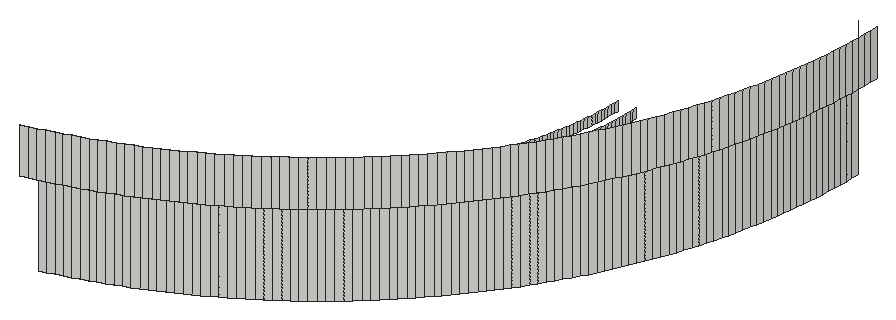
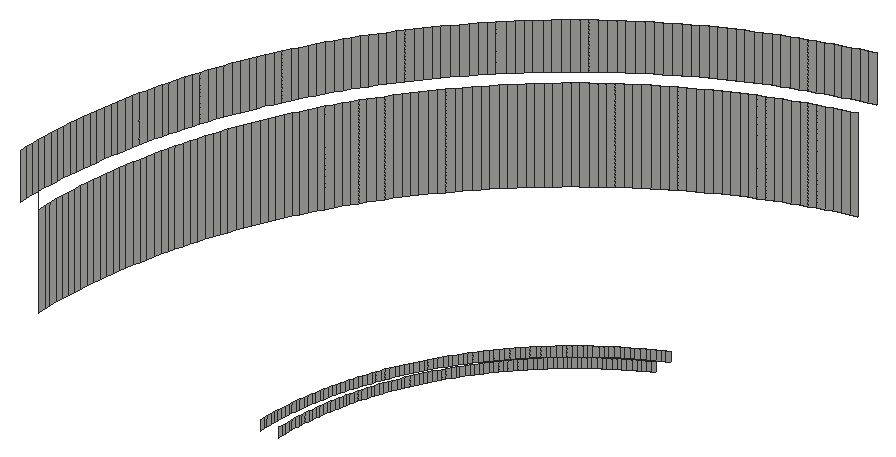
# SketchUp Ruby script. Lengths in inches.
U = 1.inch
M = Sketchup.active_model
def pt(a) = Geom::Point3d.new(a.map { |v| v * U })
def face(e, loops, mat)
  f = e.add_face(loops[0].map { |a| pt(a) })
  loops[1..].each { |l| e.add_face(l.map { |a| pt(a) }).erase! }
  f.material = f.back_material = mat if mat
  f
end
# faces: each face lists its corners as indices into pts; further lists are holes
def faces(e, pts, list, mat = nil) = list.each { |f| face(e, (f[0].is_a?(Array) ? f : [f]).map { |l| l.map { |i| pts[i] } }, mat) }
# xy, xz, yz: faces in a plane at the given z, y or x. An outline is a flat list of corners, or four numbers for a rectangle; further outlines are holes
def ring(l) = l.size == 4 ? [[l[0], l[1]], [l[2], l[1]], [l[2], l[3]], [l[0], l[3]]] : l.each_slice(2).to_a
def flat(e, list, mat, &to3) = list.each { |f| face(e, (f[0].is_a?(Array) ? f : [f]).map { |l| ring(l).map { |u, v| to3.(u, v) } }, mat) }
def xy(e, z, list, mat = nil) = flat(e, list, mat) { |x, y| [x, y, z] }
def xz(e, y, list, mat = nil) = flat(e, list, mat) { |x, z| [x, y, z] }
def yz(e, x, list, mat = nil) = flat(e, list, mat) { |y, z| [x, y, z] }
def lines(e, pts, list) = list.each { |a, b| e.add_line(pt(pts[a]), pt(pts[b])) }
# prism: a flat outline (further loops are holes) pulled along v
def prism(e, loops, v, mat = nil)
  f = face(e, loops, mat); d = Geom::Vector3d.new(v.map { |x| x * U })
  f.pushpull(f.normal.samedirection?(d) ? d.length : -d.length)
end
def box(e, o, s, mat = nil) = prism(e, [[o, [o[0] + s[0], o[1], o[2]], [o[0] + s[0], o[1] + s[1], o[2]], [o[0], o[1] + s[1], o[2]]]], [0, 0, s[2]], mat)
def at(x, y, z, deg = 0) = Geom::Transformation.translation(pt([x, y, z])) * Geom::Transformation.rotation(ORIGIN, Z_AXIS, deg.degrees)
def axes(o, x, y, z) = Geom::Transformation.new([*x, 0, *y, 0, *z, 0, *pt(o).to_a, 1])
def part(name) = M.definitions.add(name)
# library, detail: a bought-in or finely detailed component or shape, given as its bounding box
def library(name, o, s) = part(name).tap { |d| box(d.entities, o, s) }
def detail(e, o, s) = box(e.add_group.entities, o, s)
def put(e, d, t, mat = nil) = e.add_instance(d, t).tap { |i| i.material = mat if mat }
def group(e, t, mat = nil) = e.add_group.tap { |g| g.transformation = t; g.material = mat if mat }.entities
root = M.entities
yz(root,285.99,[[233.37,348,233.58,348.5]])
yz(root,286,[[233.79,348,234,348.5]])
yz(root,286.99,[[233.33,348,233.55,348.5]])
yz(root,287,[[233.78,348,234,348.5]])
yz(root,299,[[233.62,349.5,234,354.5]])
yz(root,300,[[233.61,354.5,234,357]])
p = [[277.32,218.66,348],[277.12,218.5625,348],[277.12,218.5625,348.5],[277.32,218.66,348.5],[277.52,218.75,348],[277.52,218.75,348.5],
  [277.72,218.85,348],[277.72,218.85,348.5],[277.92,218.96,348],[277.92,218.96,348.5],[278.11,219.06,348],[278.11,219.06,348.5],
  [278.31,219.17,348],[278.31,219.17,348.5],[278.5,219.28,348],[278.5,219.28,348.5],[278.69,219.39,348],[278.69,219.39,348.5],
  [278.88,219.51,348],[278.88,219.51,348.5],[279.07,219.62,348],[279.07,219.62,348.5],[279.26,219.74,348],[279.26,219.74,348.5],
  [277.08,219.65,348],[277.26,219.74,348],[277.26,219.74,348.5],[277.08,219.65,348.5],[277.45,219.84,348],[277.45,219.84,348.5],
  [279.44,219.87,348],[279.44,219.87,348.5],[277.63,219.9375,348],[277.63,219.9375,348.5],[277.82,220.04,348],[277.82,220.04,348.5],
  [279.63,219.99,348],[279.63,219.99,348.5],[278,220.14,348],[278,220.14,348.5],[279.8125,220.12,348],[279.8125,220.12,348.5],
  [278.18,220.25,348],[278.18,220.25,348.5],[279.99,220.25,348],[279.99,220.25,348.5],[278.36,220.36,348],[278.36,220.36,348.5],
  [280.17,220.38,348],[280.17,220.38,348.5],[278.54,220.47,348],[278.54,220.47,348.5],[280.35,220.51,348],[280.35,220.51,348.5],
  [278.71,220.58,348],[278.71,220.58,348.5],[280.52,220.65,348],[280.52,220.65,348.5],[278.89,220.7,348],[278.89,220.7,348.5],
  [280.7,220.79,348],[280.7,220.79,348.5],[279.0625,220.8125,348],[279.0625,220.8125,348.5],[279.23,220.93,348],[279.23,220.93,348.5],
  [280.87,220.93,348],[280.87,220.93,348.5],[279.4,221.06,348],[279.4,221.06,348.5],[281.04,221.07,348],[281.04,221.07,348.5],
  [279.57,221.18,348],[279.57,221.18,348.5],[281.21,221.22,348],[281.21,221.22,348.5],[279.74,221.31,348],[279.74,221.31,348.5],
  [281.375,221.37,348],[281.375,221.37,348.5],[279.91,221.43,348],[279.91,221.43,348.5],[280.07,221.57,348],[280.07,221.57,348.5],
  [281.54,221.52,348],[281.54,221.52,348.5],[281.7,221.67,348],[281.7,221.67,348.5],[280.23,221.7,348],[280.23,221.7,348.5],
  [280.39,221.83,348],[280.39,221.83,348.5],[281.86,221.82,348],[281.86,221.82,348.5],[280.55,221.97,348],[280.55,221.97,348.5],
  [282.02,221.98,348],[282.02,221.98,348.5],[280.71,222.11,348],[280.71,222.11,348.5],[282.18,222.14,348],[282.18,222.14,348.5],
  [280.86,222.25,348],[280.86,222.25,348.5],[282.33,222.3,348],[282.33,222.3,348.5],[281.01,222.39,348],[281.01,222.39,348.5],
  [282.48,222.46,348],[282.48,222.46,348.5],[281.16,222.54,348],[281.16,222.54,348.5],[281.3125,222.6875,348],[281.3125,222.6875,348.5],
  [282.63,222.625,348],[282.63,222.625,348.5],[282.78,222.79,348],[282.78,222.79,348.5],[281.46,222.84,348],[281.46,222.84,348.5],
  [281.61,222.99,348],[281.61,222.99,348.5],[282.93,222.96,348],[282.93,222.96,348.5],[281.75,223.14,348],[281.75,223.14,348.5],
  [283.07,223.13,348],[283.07,223.13,348.5],[281.89,223.29,348],[281.89,223.29,348.5],[283.21,223.3,348],[283.21,223.3,348.5],
  [282.03,223.45,348],[282.03,223.45,348.5],[283.35,223.48,348],[283.35,223.48,348.5],[282.17,223.61,348],[282.17,223.61,348.5],
  [283.49,223.65,348],[283.49,223.65,348.5],[282.3,223.77,348],[282.3,223.77,348.5],[283.62,223.83,348],[283.62,223.83,348.5],
  [282.43,223.93,348],[282.43,223.93,348.5],[283.75,224.01,348],[283.75,224.01,348.5],[282.57,224.09,348],[282.57,224.09,348.5],
  [283.88,224.1875,348],[283.88,224.1875,348.5],[282.69,224.26,348],[282.69,224.26,348.5],[284.01,224.37,348],[284.01,224.37,348.5],
  [282.82,224.43,348],[282.82,224.43,348.5],[282.94,224.6,348],[282.94,224.6,348.5],[284.13,224.56,348],[284.13,224.56,348.5],
  [283.07,224.77,348],[283.07,224.77,348.5],[284.26,224.74,348],[284.26,224.74,348.5],[284.38,224.93,348],[284.38,224.93,348.5],
  [283.1875,224.9375,348],[283.1875,224.9375,348.5],[283.3,225.11,348],[283.3,225.11,348.5],[284.49,225.12,348],[284.49,225.12,348.5],
  [283.42,225.29,348],[283.42,225.29,348.5],[284.61,225.31,348],[284.61,225.31,348.5],[283.53,225.46,348],[283.53,225.46,348.5],
  [284.72,225.5,348],[284.72,225.5,348.5],[283.64,225.64,348],[283.64,225.64,348.5],[284.83,225.69,348],[284.83,225.69,348.5],
  [283.75,225.82,348],[283.75,225.82,348.5],[284.94,225.89,348],[284.94,225.89,348.5],[283.86,226,348],[283.86,226,348.5],
  [285.04,226.08,348],[285.04,226.08,348.5],[283.96,226.18,348],[283.96,226.18,348.5],[285.15,226.28,348],[285.15,226.28,348.5],
  [284.0625,226.37,348],[284.0625,226.37,348.5],[285.25,226.48,348],[285.25,226.48,348.5],[284.16,226.55,348],[284.16,226.55,348.5],
  [285.34,226.68,348],[285.34,226.68,348.5],[284.26,226.74,348],[284.26,226.74,348.5],[284.35,226.92,348],[284.35,226.92,348.5],
  [285.4375,226.88,348],[285.4375,226.88,348.5],[284.44,227.11,348],[284.44,227.11,348.5],[285.53,227.09,348],[285.53,227.09,348.5],
  [284.53,227.3,348],[284.53,227.3,348.5],[285.62,227.29,348],[285.62,227.29,348.5],[284.62,227.49,348],[284.62,227.49,348.5],
  [285.71,227.49,348],[285.71,227.49,348.5],[284.7,227.68,348],[284.7,227.68,348.5],[285.79,227.7,348],[285.79,227.7,348.5],
  [284.78,227.88,348],[284.78,227.88,348.5],[285.87,227.91,348],[285.87,227.91,348.5],[284.86,228.07,348],[284.86,228.07,348.5],
  [285.95,228.12,348],[285.95,228.12,348.5],[284.9375,228.27,348],[284.9375,228.27,348.5],[286.02,228.33,348],[286.02,228.33,348.5],
  [285.01,228.46,348],[285.01,228.46,348.5],[286.1,228.54,348],[286.1,228.54,348.5],[285.08,228.66,348],[285.08,228.66,348.5],
  [286.17,228.75,348],[286.17,228.75,348.5],[285.15,228.86,348],[285.15,228.86,348.5],[286.24,228.96,348],[286.24,228.96,348.5],
  [285.22,229.06,348],[285.22,229.06,348.5],[286.3,229.17,348],[286.3,229.17,348.5],[285.28,229.26,348],[285.28,229.26,348.5],
  [286.36,229.39,348],[286.36,229.39,348.5],[285.34,229.46,348],[285.34,229.46,348.5],[286.42,229.6,348],[286.42,229.6,348.5],
  [285.4,229.66,348],[285.4,229.66,348.5],[286.48,229.82,348],[286.48,229.82,348.5],[285.45,229.86,348],[285.45,229.86,348.5],
  [286.53,230.03,348],[286.53,230.03,348.5],[285.51,230.0625,348],[285.51,230.0625,348.5],[286.58,230.25,348],[286.58,230.25,348.5],
  [285.56,230.26,348],[285.56,230.26,348.5],[286.63,230.47,348],[286.63,230.47,348.5],[285.61,230.47,348],[285.61,230.47,348.5],
  [285.65,230.67,348],[285.65,230.67,348.5],[286.67,230.68,348],[286.67,230.68,348.5],[285.69,230.88,348],[285.69,230.88,348.5],
  [286.72,230.9,348],[286.72,230.9,348.5],[285.73,231.08,348],[285.73,231.08,348.5],[286.75,231.12,348],[286.75,231.12,348.5],
  [285.77,231.29,348],[285.77,231.29,348.5],[286.79,231.34,348],[286.79,231.34,348.5],[285.8,231.5,348],[285.8,231.5,348.5],
  [286.82,231.5625,348],[286.82,231.5625,348.5],[285.83,231.7,348],[285.83,231.7,348.5],[286.85,231.78,348],[286.85,231.78,348.5],
  [285.86,231.91,348],[285.86,231.91,348.5],[286.88,232,348],[286.88,232,348.5],[285.89,232.12,348],[285.89,232.12,348.5],
  [286.91,232.22,348],[286.91,232.22,348.5],[285.91,232.33,348],[285.91,232.33,348.5],[286.93,232.44,348],[286.93,232.44,348.5],
  [285.93,232.54,348],[285.93,232.54,348.5],[286.95,232.67,348],[286.95,232.67,348.5],[285.95,232.74,348],[285.95,232.74,348.5],
  [285.97,232.95,348],[285.97,232.95,348.5],[286.96,232.89,348],[286.96,232.89,348.5],[286.98,233.11,348],[286.98,233.11,348.5],
  [285.98,233.16,348],[285.98,233.16,348.5],[286.99,233.33,348],[286.99,233.33,348.5],[285.99,233.37,348],[285.99,233.37,348.5],
  [285.99,233.58,348],[286,233.79,348],[286,233.79,348.5],[285.99,233.58,348.5],[287,233.78,348],[286.99,233.55,348],
  [286.99,233.55,348.5],[287,233.78,348.5],[277.14,205.89,349.5],[277.51,205.99,349.5],[277.51,205.99,354.5],[277.14,205.89,354.5],
  [277.87,206.09,349.5],[277.87,206.09,354.5],[278.24,206.19,349.5],[278.24,206.19,354.5],[278.6,206.3,349.5],[278.6,206.3,354.5],
  [278.96,206.42,349.5],[278.96,206.42,354.5],[279.32,206.54,349.5],[279.32,206.54,354.5],[279.68,206.66,349.5],[279.68,206.66,354.5],
  [280.04,206.79,349.5],[280.04,206.79,354.5],[280.39,206.93,349.5],[280.39,206.93,354.5],[280.75,207.06,349.5],[280.75,207.06,354.5],
  [281.1,207.21,349.5],[281.1,207.21,354.5],[281.45,207.36,349.5],[281.45,207.36,354.5],[281.8,207.51,349.5],[281.8,207.51,354.5],
  [282.14,207.66,349.5],[282.14,207.66,354.5],[282.48,207.83,349.5],[282.48,207.83,354.5],[282.83,207.99,349.5],[282.83,207.99,354.5],
  [283.17,208.16,349.5],[283.17,208.16,354.5],[283.5,208.34,349.5],[283.5,208.34,354.5],[283.84,208.51,349.5],[283.84,208.51,354.5],
  [284.17,208.7,349.5],[284.17,208.7,354.5],[284.5,208.89,349.5],[284.5,208.89,354.5],[284.83,209.08,349.5],[284.83,209.08,354.5],
  [285.15,209.27,349.5],[285.15,209.27,354.5],[285.47,209.47,349.5],[285.47,209.47,354.5],[285.79,209.68,349.5],[285.79,209.68,354.5],
  [286.11,209.89,349.5],[286.11,209.89,354.5],[286.43,210.1,349.5],[286.43,210.1,354.5],[286.74,210.32,349.5],[286.74,210.32,354.5],
  [287.05,210.54,349.5],[287.05,210.54,354.5],[287.35,210.76,349.5],[287.35,210.76,354.5],[287.65,210.99,349.5],[287.65,210.99,354.5],
  [287.95,211.23,349.5],[287.95,211.23,354.5],[288.25,211.46,349.5],[288.25,211.46,354.5],[288.54,211.7,349.5],[288.54,211.7,354.5],
  [288.83,211.95,349.5],[288.83,211.95,354.5],[289.12,212.2,349.5],[289.12,212.2,354.5],[289.4,212.45,349.5],[289.4,212.45,354.5],
  [289.69,212.7,349.5],[289.69,212.7,354.5],[289.96,212.96,349.5],[289.96,212.96,354.5],[290.24,213.23,349.5],[290.24,213.23,354.5],
  [290.51,213.49,349.5],[290.51,213.49,354.5],[290.77,213.76,349.5],[290.77,213.76,354.5],[291.04,214.04,349.5],[291.04,214.04,354.5],
  [291.3,214.31,349.5],[291.3,214.31,354.5],[291.55,214.6,349.5],[291.55,214.6,354.5],[291.8,214.88,349.5],[291.8,214.88,354.5],
  [292.05,215.17,349.5],[292.05,215.17,354.5],[292.3,215.46,349.5],[292.3,215.46,354.5],[292.54,215.75,349.5],[292.54,215.75,354.5],
  [292.77,216.05,349.5],[292.77,216.05,354.5],[293.01,216.35,349.5],[293.01,216.35,354.5],[293.24,216.65,349.5],[293.24,216.65,354.5],
  [293.46,216.95,349.5],[293.46,216.95,354.5],[293.68,217.26,349.5],[293.68,217.26,354.5],[293.9,217.57,349.5],[293.9,217.57,354.5],
  [294.11,217.89,349.5],[294.11,217.89,354.5],[294.32,218.21,349.5],[294.32,218.21,354.5],[294.53,218.53,349.5],[294.53,218.53,354.5],
  [294.73,218.85,349.5],[294.73,218.85,354.5],[294.92,219.17,349.5],[294.92,219.17,354.5],[295.11,219.5,349.5],[295.11,219.5,354.5],
  [295.3,219.83,349.5],[295.3,219.83,354.5],[295.49,220.16,349.5],[295.49,220.16,354.5],[295.66,220.5,349.5],[295.66,220.5,354.5],
  [295.84,220.83,349.5],[295.84,220.83,354.5],[296.01,221.17,349.5],[296.01,221.17,354.5],[296.17,221.52,349.5],[296.17,221.52,354.5],
  [296.34,221.86,349.5],[296.34,221.86,354.5],[296.49,222.2,349.5],[296.49,222.2,354.5],[296.64,222.55,349.5],[296.64,222.55,354.5],
  [296.79,222.9,349.5],[296.79,222.9,354.5],[296.94,223.25,349.5],[296.94,223.25,354.5],[297.07,223.61,349.5],[297.07,223.61,354.5],
  [297.21,223.96,349.5],[297.21,223.96,354.5],[297.34,224.32,349.5],[297.34,224.32,354.5],[297.46,224.68,349.5],[297.46,224.68,354.5],
  [297.58,225.04,349.5],[297.58,225.04,354.5],[297.7,225.4,349.5],[297.7,225.4,354.5],[297.81,225.76,349.5],[297.81,225.76,354.5],
  [297.91,226.13,349.5],[297.91,226.13,354.5],[298.01,226.49,349.5],[298.01,226.49,354.5],[298.11,226.86,349.5],[298.11,226.86,354.5],
  [298.2,227.23,349.5],[298.2,227.23,354.5],[298.28,227.6,349.5],[298.28,227.6,354.5],[298.37,227.97,349.5],[298.37,227.97,354.5],
  [298.44,228.34,349.5],[298.44,228.34,354.5],[298.51,228.72,349.5],[298.51,228.72,354.5],[298.58,229.09,349.5],[298.58,229.09,354.5],
  [298.64,229.46,349.5],[298.64,229.46,354.5],[298.7,229.84,349.5],[298.7,229.84,354.5],[298.75,230.21,349.5],[298.75,230.21,354.5],
  [298.8,230.59,349.5],[298.8,230.59,354.5],[298.84,230.97,349.5],[298.84,230.97,354.5],[298.88,231.35,349.5],[298.88,231.35,354.5],
  [298.91,231.72,349.5],[298.91,231.72,354.5],[298.9375,232.1,349.5],[298.9375,232.1,354.5],[298.96,232.48,349.5],[298.96,232.48,354.5],
  [298.98,232.86,349.5],[298.98,232.86,354.5],[298.99,233.24,349.5],[298.99,233.24,354.5],[299,233.62,349.5],[299,233.62,354.5],
  [277,204.83,354.5],[277.38,204.92,354.5],[277.38,204.92,357],[277,204.83,357],[277.76,205.02,354.5],[277.76,205.02,357],
  [278.14,205.125,354.5],[278.14,205.125,357],[278.52,205.24,354.5],[278.52,205.24,357],[278.9,205.35,354.5],[278.9,205.35,357],
  [279.27,205.47,354.5],[279.27,205.47,357],[279.64,205.59,354.5],[279.64,205.59,357],[280.01,205.72,354.5],[280.01,205.72,357],
  [280.38,205.85,354.5],[280.38,205.85,357],[280.75,205.99,354.5],[280.75,205.99,357],[281.12,206.14,354.5],[281.12,206.14,357],
  [281.48,206.28,354.5],[281.48,206.28,357],[281.84,206.4375,354.5],[281.84,206.4375,357],[282.2,206.59,354.5],[282.2,206.59,357],
  [282.56,206.76,354.5],[282.56,206.76,357],[282.92,206.92,354.5],[282.92,206.92,357],[283.27,207.09,354.5],[283.27,207.09,357],
  [283.62,207.27,354.5],[283.62,207.27,357],[283.97,207.45,354.5],[283.97,207.45,357],[284.31,207.64,354.5],[284.31,207.64,357],
  [284.66,207.83,354.5],[284.66,207.83,357],[285,208.02,354.5],[285,208.02,357],[285.34,208.22,354.5],[285.34,208.22,357],
  [285.67,208.42,354.5],[285.67,208.42,357],[286.01,208.63,354.5],[286.01,208.63,357],[286.34,208.84,354.5],[286.34,208.84,357],
  [286.67,209.06,354.5],[286.67,209.06,357],[286.99,209.28,354.5],[286.99,209.28,357],[287.3125,209.5,354.5],[287.3125,209.5,357],
  [287.63,209.73,354.5],[287.63,209.73,357],[287.95,209.96,354.5],[287.95,209.96,357],[288.26,210.2,354.5],[288.26,210.2,357],
  [288.57,210.44,354.5],[288.57,210.44,357],[288.88,210.6875,354.5],[288.88,210.6875,357],[289.18,210.93,354.5],[289.18,210.93,357],
  [289.48,211.1875,354.5],[289.48,211.1875,357],[289.78,211.44,354.5],[289.78,211.44,357],[290.07,211.71,354.5],[290.07,211.71,357],
  [290.36,211.97,354.5],[290.36,211.97,357],[290.65,212.24,354.5],[290.65,212.24,357],[290.93,212.51,354.5],[290.93,212.51,357],
  [291.21,212.79,354.5],[291.21,212.79,357],[291.49,213.07,354.5],[291.49,213.07,357],[291.76,213.35,354.5],[291.76,213.35,357],
  [292.03,213.64,354.5],[292.03,213.64,357],[292.29,213.93,354.5],[292.29,213.93,357],[292.56,214.22,354.5],[292.56,214.22,357],
  [292.8125,214.52,354.5],[292.8125,214.52,357],[293.07,214.82,354.5],[293.07,214.82,357],[293.3125,215.12,354.5],[293.3125,215.12,357],
  [293.56,215.43,354.5],[293.56,215.43,357],[293.8,215.74,354.5],[293.8,215.74,357],[294.04,216.05,354.5],[294.04,216.05,357],
  [294.27,216.37,354.5],[294.27,216.37,357],[294.5,216.6875,354.5],[294.5,216.6875,357],[294.72,217.01,354.5],[294.72,217.01,357],
  [294.94,217.33,354.5],[294.94,217.33,357],[295.16,217.66,354.5],[295.16,217.66,357],[295.37,217.99,354.5],[295.37,217.99,357],
  [295.58,218.33,354.5],[295.58,218.33,357],[295.78,218.66,354.5],[295.78,218.66,357],[295.98,219,354.5],[295.98,219,357],
  [296.17,219.34,354.5],[296.17,219.34,357],[296.36,219.69,354.5],[296.36,219.69,357],[296.55,220.03,354.5],[296.55,220.03,357],
  [296.73,220.38,354.5],[296.73,220.38,357],[296.91,220.73,354.5],[296.91,220.73,357],[297.08,221.08,354.5],[297.08,221.08,357],
  [297.24,221.44,354.5],[297.24,221.44,357],[297.41,221.8,354.5],[297.41,221.8,357],[297.5625,222.16,354.5],[297.5625,222.16,357],
  [297.72,222.52,354.5],[297.72,222.52,357],[297.86,222.88,354.5],[297.86,222.88,357],[298.01,223.25,354.5],[298.01,223.25,357],
  [298.15,223.62,354.5],[298.15,223.62,357],[298.28,223.99,354.5],[298.28,223.99,357],[298.41,224.36,354.5],[298.41,224.36,357],
  [298.53,224.73,354.5],[298.53,224.73,357],[298.65,225.1,354.5],[298.65,225.1,357],[298.76,225.48,354.5],[298.76,225.48,357],
  [298.875,225.86,354.5],[298.875,225.86,357],[298.98,226.24,354.5],[298.98,226.24,357],[299.08,226.62,354.5],[299.08,226.62,357],
  [299.17,227,354.5],[299.17,227,357],[299.26,227.38,354.5],[299.26,227.38,357],[299.34,227.76,354.5],[299.34,227.76,357],
  [299.42,228.15,354.5],[299.42,228.15,357],[299.5,228.53,354.5],[299.5,228.53,357],[299.57,228.92,354.5],[299.57,228.92,357],
  [299.63,229.31,354.5],[299.63,229.31,357],[299.69,229.7,354.5],[299.69,229.7,357],[299.74,230.08,354.5],[299.74,230.08,357],
  [299.79,230.47,354.5],[299.79,230.47,357],[299.84,230.86,354.5],[299.84,230.86,357],[299.875,231.25,354.5],[299.875,231.25,357],
  [299.91,231.65,354.5],[299.91,231.65,357],[299.9375,232.04,354.5],[299.9375,232.04,357],[299.96,232.43,354.5],[299.96,232.43,357],
  [299.98,232.82,354.5],[299.98,232.82,357],[299.99,233.21,354.5],[299.99,233.21,357],[300,233.61,354.5],[300,233.61,357],
  [299,234,354.5],[299,234,357]]
faces(root,p,[[0,1,2,3],[4,0,3,5],[6,4,5,7],[8,6,7,9],[10,8,9,11],[12,10,11,13],[14,12,13,15],[16,14,15,17],
  [18,16,17,19],[20,18,19,21],[22,20,21,23],[24,25,26,27],[25,28,29,26],[30,22,23,31],[28,32,33,29],[32,34,35,33],
  [36,30,31,37],[34,38,39,35],[40,36,37,41],[38,42,43,39],[44,40,41,45],[42,46,47,43],[48,44,45,49],[46,50,51,47],
  [52,48,49,53],[50,54,55,51],[56,52,53,57],[54,58,59,55],[60,56,57,61],[58,62,63,59],[62,64,65,63],[66,60,61,67],
  [64,68,69,65],[70,66,67,71],[68,72,73,69],[74,70,71,75],[72,76,77,73],[78,74,75,79],[76,80,81,77],[80,82,83,81],
  [84,78,79,85],[86,84,85,87],[82,88,89,83],[88,90,91,89],[92,86,87,93],[90,94,95,91],[96,92,93,97],[94,98,99,95],
  [100,96,97,101],[98,102,103,99],[104,100,101,105],[102,106,107,103],[108,104,105,109],[106,110,111,107],[110,112,113,111],[114,108,109,115],
  [116,114,115,117],[112,118,119,113],[118,120,121,119],[122,116,117,123],[120,124,125,121],[126,122,123,127],[124,128,129,125],[130,126,127,131],
  [128,132,133,129],[134,130,131,135],[132,136,137,133],[138,134,135,139],[136,140,141,137],[142,138,139,143],[140,144,145,141],[146,142,143,147],
  [144,148,149,145],[150,146,147,151],[148,152,153,149],[154,150,151,155],[152,156,157,153],[156,158,159,157],[160,154,155,161],[158,162,163,159],
  [164,160,161,165],[166,164,165,167],[162,168,169,163],[168,170,171,169],[172,166,167,173],[170,174,175,171],[176,172,173,177],[174,178,179,175],
  [180,176,177,181],[178,182,183,179],[184,180,181,185],[182,186,187,183],[188,184,185,189],[186,190,191,187],[192,188,189,193],[190,194,195,191],
  [196,192,193,197],[194,198,199,195],[200,196,197,201],[198,202,203,199],[204,200,201,205],[202,206,207,203],[206,208,209,207],[210,204,205,211],
  [208,212,213,209],[214,210,211,215],[212,216,217,213],[218,214,215,219],[216,220,221,217],[222,218,219,223],[220,224,225,221],[226,222,223,227],
  [224,228,229,225],[230,226,227,231],[228,232,233,229],[234,230,231,235],[232,236,237,233],[238,234,235,239],[236,240,241,237],[242,238,239,243],
  [240,244,245,241],[246,242,243,247],[244,248,249,245],[250,246,247,251],[248,252,253,249],[254,250,251,255],[252,256,257,253],[258,254,255,259],
  [256,260,261,257],[262,258,259,263],[260,264,265,261],[266,262,263,267],[264,268,269,265],[270,266,267,271],[268,272,273,269],[274,270,271,275],
  [272,276,277,273],[278,274,275,279],[276,280,281,277],[280,282,283,281],[284,278,279,285],[282,286,287,283],[288,284,285,289],[286,290,291,287],
  [292,288,289,293],[290,294,295,291],[296,292,293,297],[294,298,299,295],[300,296,297,301],[298,302,303,299],[304,300,301,305],[302,306,307,303],
  [308,304,305,309],[306,310,311,307],[312,308,309,313],[310,314,315,311],[316,312,313,317],[314,318,319,315],[320,316,317,321],[318,322,323,319],
  [322,324,325,323],[326,320,321,327],[328,326,327,329],[324,330,331,325],[332,328,329,333],[330,334,335,331],[336,337,338,339],[340,341,342,343],
  [344,345,346,347],[345,348,349,346],[348,350,351,349],[350,352,353,351],[352,354,355,353],[354,356,357,355],[356,358,359,357],[358,360,361,359],
  [360,362,363,361],[362,364,365,363],[364,366,367,365],[366,368,369,367],[368,370,371,369],[370,372,373,371],[372,374,375,373],[374,376,377,375],
  [376,378,379,377],[378,380,381,379],[380,382,383,381],[382,384,385,383],[384,386,387,385],[386,388,389,387],[388,390,391,389],[390,392,393,391],
  [392,394,395,393],[394,396,397,395],[396,398,399,397],[398,400,401,399],[400,402,403,401],[402,404,405,403],[404,406,407,405],[406,408,409,407],
  [408,410,411,409],[410,412,413,411],[412,414,415,413],[414,416,417,415],[416,418,419,417],[418,420,421,419],[420,422,423,421],[422,424,425,423],
  [424,426,427,425],[426,428,429,427],[428,430,431,429],[430,432,433,431],[432,434,435,433],[434,436,437,435],[436,438,439,437],[438,440,441,439],
  [440,442,443,441],[442,444,445,443],[444,446,447,445],[446,448,449,447],[448,450,451,449],[450,452,453,451],[452,454,455,453],[454,456,457,455],
  [456,458,459,457],[458,460,461,459],[460,462,463,461],[462,464,465,463],[464,466,467,465],[466,468,469,467],[468,470,471,469],[470,472,473,471],
  [472,474,475,473],[474,476,477,475],[476,478,479,477],[478,480,481,479],[480,482,483,481],[482,484,485,483],[484,486,487,485],[486,488,489,487],
  [488,490,491,489],[490,492,493,491],[492,494,495,493],[494,496,497,495],[496,498,499,497],[498,500,501,499],[500,502,503,501],[502,504,505,503],
  [504,506,507,505],[506,508,509,507],[508,510,511,509],[510,512,513,511],[512,514,515,513],[514,516,517,515],[516,518,519,517],[518,520,521,519],
  [520,522,523,521],[522,524,525,523],[524,526,527,525],[526,528,529,527],[528,530,531,529],[530,532,533,531],[532,534,535,533],[534,536,537,535],
  [536,538,539,537],[538,540,541,539],[540,542,543,541],[542,544,545,543],[546,547,548,549],[547,550,551,548],[550,552,553,551],[552,554,555,553],
  [554,556,557,555],[556,558,559,557],[558,560,561,559],[560,562,563,561],[562,564,565,563],[564,566,567,565],[566,568,569,567],[568,570,571,569],
  [570,572,573,571],[572,574,575,573],[574,576,577,575],[576,578,579,577],[578,580,581,579],[580,582,583,581],[582,584,585,583],[584,586,587,585],
  [586,588,589,587],[588,590,591,589],[590,592,593,591],[592,594,595,593],[594,596,597,595],[596,598,599,597],[598,600,601,599],[600,602,603,601],
  [602,604,605,603],[604,606,607,605],[606,608,609,607],[608,610,611,609],[610,612,613,611],[612,614,615,613],[614,616,617,615],[616,618,619,617],
  [618,620,621,619],[620,622,623,621],[622,624,625,623],[624,626,627,625],[626,628,629,627],[628,630,631,629],[630,632,633,631],[632,634,635,633],
  [634,636,637,635],[636,638,639,637],[638,640,641,639],[640,642,643,641],[642,644,645,643],[644,646,647,645],[646,648,649,647],[648,650,651,649],
  [650,652,653,651],[652,654,655,653],[654,656,657,655],[656,658,659,657],[658,660,661,659],[660,662,663,661],[662,664,665,663],[664,666,667,665],
  [666,668,669,667],[668,670,671,669],[670,672,673,671],[672,674,675,673],[674,676,677,675],[676,678,679,677],[678,680,681,679],[680,682,683,681],
  [682,684,685,683],[684,686,687,685],[686,688,689,687],[688,690,691,689],[690,692,693,691],[692,694,695,693],[694,696,697,695],[696,698,699,697],
  [698,700,701,699],[700,702,703,701],[702,704,705,703],[704,706,707,705],[706,708,709,707],[708,710,711,709],[710,712,713,711],[712,714,715,713],
  [714,716,717,715],[716,718,719,717],[718,720,721,719],[720,722,723,721],[722,724,725,723],[724,726,727,725],[726,728,729,727],[728,730,731,729],
  [730,732,733,731],[732,734,735,733],[734,736,737,735],[736,738,739,737],[738,740,741,739],[740,742,743,741],[742,744,745,743],[744,746,747,745],
  [746,748,749,747]])
lines(root,p,[[750,751]])
